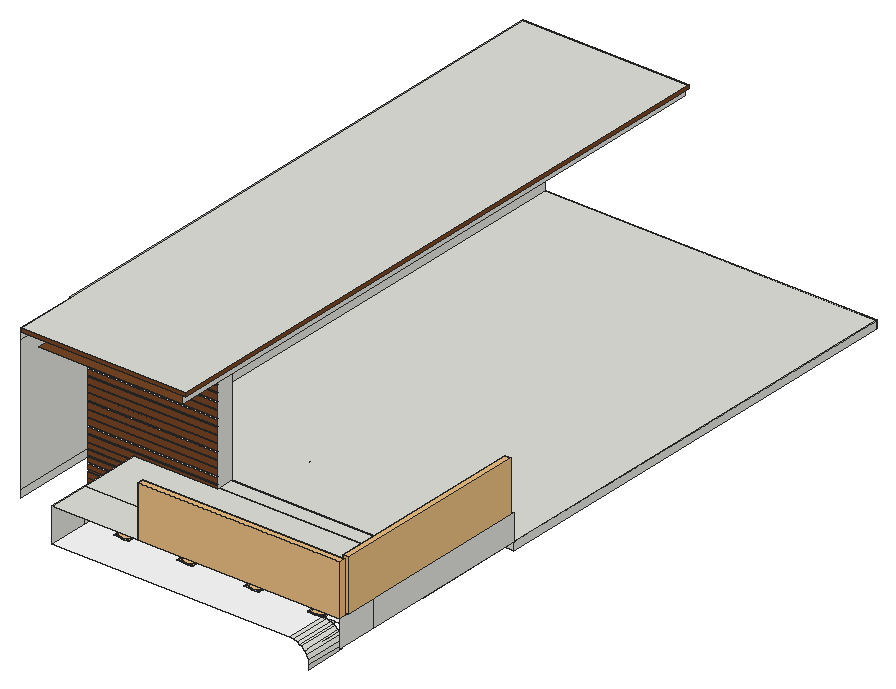
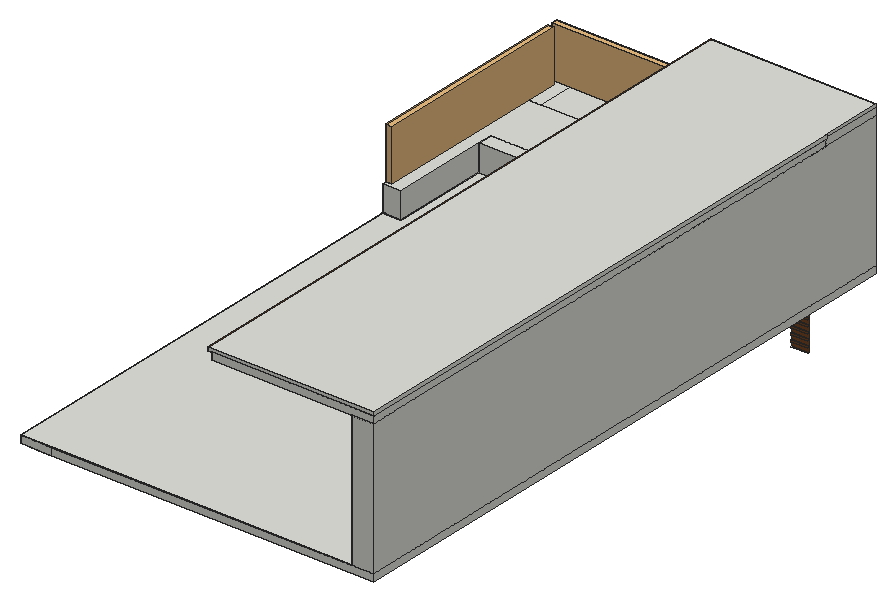
# SketchUp Ruby script. Lengths in inches.
U = 1.inch
M = Sketchup.active_model
def pt(a) = Geom::Point3d.new(a.map { |v| v * U })
def face(e, loops, mat)
  f = e.add_face(loops[0].map { |a| pt(a) })
  loops[1..].each { |l| e.add_face(l.map { |a| pt(a) }).erase! }
  f.material = f.back_material = mat if mat
  f
end
# faces: each face lists its corners as indices into pts; further lists are holes
def faces(e, pts, list, mat = nil) = list.each { |f| face(e, (f[0].is_a?(Array) ? f : [f]).map { |l| l.map { |i| pts[i] } }, mat) }
# xy, xz, yz: faces in a plane at the given z, y or x. An outline is a flat list of corners, or four numbers for a rectangle; further outlines are holes
def ring(l) = l.size == 4 ? [[l[0], l[1]], [l[2], l[1]], [l[2], l[3]], [l[0], l[3]]] : l.each_slice(2).to_a
def flat(e, list, mat, &to3) = list.each { |f| face(e, (f[0].is_a?(Array) ? f : [f]).map { |l| ring(l).map { |u, v| to3.(u, v) } }, mat) }
def xy(e, z, list, mat = nil) = flat(e, list, mat) { |x, y| [x, y, z] }
def xz(e, y, list, mat = nil) = flat(e, list, mat) { |x, z| [x, y, z] }
def yz(e, x, list, mat = nil) = flat(e, list, mat) { |y, z| [x, y, z] }
def lines(e, pts, list) = list.each { |a, b| e.add_line(pt(pts[a]), pt(pts[b])) }
# prism: a flat outline (further loops are holes) pulled along v
def prism(e, loops, v, mat = nil)
  f = face(e, loops, mat); d = Geom::Vector3d.new(v.map { |x| x * U })
  f.pushpull(f.normal.samedirection?(d) ? d.length : -d.length)
end
def box(e, o, s, mat = nil) = prism(e, [[o, [o[0] + s[0], o[1], o[2]], [o[0] + s[0], o[1] + s[1], o[2]], [o[0], o[1] + s[1], o[2]]]], [0, 0, s[2]], mat)
def at(x, y, z, deg = 0) = Geom::Transformation.translation(pt([x, y, z])) * Geom::Transformation.rotation(ORIGIN, Z_AXIS, deg.degrees)
def axes(o, x, y, z) = Geom::Transformation.new([*x, 0, *y, 0, *z, 0, *pt(o).to_a, 1])
def part(name) = M.definitions.add(name)
# library, detail: a bought-in or finely detailed component or shape, given as its bounding box
def library(name, o, s) = part(name).tap { |d| box(d.entities, o, s) }
def detail(e, o, s) = box(e.add_group.entities, o, s)
def put(e, d, t, mat = nil) = e.add_instance(d, t).tap { |i| i.material = mat if mat }
def group(e, t, mat = nil) = e.add_group.tap { |g| g.transformation = t; g.material = mat if mat }.entities
root = M.entities
M.materials.add("[Color M00]").color = [255, 255, 255]
M.materials.add("[Wood Veneer 01]").color = [120, 70, 37]
c1 = library("Group\#12",[-0.5,-0.5,-0.1],[12.57,12.57,0.2])
c2 = library("Group\#13",[-0.5,-0.5,-0.1],[12.57,12.57,0.2])
c3 = library("Group\#14",[-0.5,-0.5,-0.1],[12.57,12.57,0.2])
c4 = library("Group\#15",[-0.5,-0.5,-0.1],[12.57,12.57,0.2])
c5 = library("Glass Railing",[0,0,0],[139.5,4.76,42])
c6 = library("Group\#8",[-0.5,-0.5,-0.1],[8.875,8.875,0.2])
c7 = library("Group\#9",[-0.5,-0.5,-0.1],[8.875,8.875,0.2])
c8 = library("Group\#11",[-0.5,-0.5,-0.1],[8.875,8.875,0.2])
xy(root,277.97,[[404.9375,346.73,445.11,348.1]])
xy(root,278.29,[[338.58,346.73,352.5,348.1]])
xy(root,281.74,[[404.9375,346.73,445.11,348.1]])
xy(root,282.01,[[338.58,346.73,352.5,348.1]])
xy(root,283.15,[[404.9375,346.73,445.11,348.1]])
xy(root,283.42,[[338.58,346.73,352.5,348.1]])
xy(root,286.91,[[404.9375,346.73,445.11,348.1]])
xy(root,287.14,[[338.58,346.73,352.5,348.1]])
xy(root,288.33,[[404.9375,346.73,445.11,348.1]])
xy(root,288.56,[[338.58,346.73,352.5,348.1]])
xy(root,292.09,[[404.9375,346.73,445.11,348.1]])
xy(root,292.28,[[338.58,346.73,352.5,348.1]])
xy(root,293.51,[[404.9375,346.73,445.11,348.1]])
xy(root,293.6875,[[338.58,346.73,352.5,348.1]])
xy(root,296,[[479.29,440.43,567.52,449.58]])
xy(root,297.27,[[404.9375,346.73,445.11,348.1]])
xy(root,297.41,[[338.58,346.73,352.5,348.1]])
xy(root,298.69,[[404.9375,346.73,445.11,348.1]])
xy(root,298.82,[[338.58,346.73,352.5,348.1]])
xy(root,302.45,[[404.9375,346.73,445.11,348.1]])
xy(root,302.54,[[338.58,346.73,352.5,348.1]])
xy(root,303.86,[[404.9375,346.73,445.11,348.1]])
xy(root,303.96,[[338.58,346.73,352.5,348.1]])
xy(root,307.63,[[404.9375,346.73,445.11,348.1]])
xy(root,307.68,[[338.58,346.73,352.5,348.1]])
xy(root,309.04,[[404.9375,346.73,445.11,348.1]])
xy(root,309.09,[[338.58,346.73,352.5,348.1]])
xy(root,312.81,[[338.58,346.73,352.5,348.1],[404.9375,346.73,445.11,348.1],[352.5,348.1,404.9375,354.42]])
xy(root,314.22,[[338.58,346.73,445.11,348.1]])
xy(root,317.66,[[376.54,346.73,445.11,348.1]])
xy(root,319.25,[[588.04,296.73,597.79,348.1],[588.04,348.1,597.79,440.43],[338.58,355.13,338.58,804.07,567.52,804.07,567.52,449.58,432.33,449.58,432.33,355.13],[338.58,355.13,338.58,804.07,567.52,804.07,567.52,449.58,432.33,449.58,432.33,355.13],[586.74,440.43,597.79,811.1],
  [597.79,440.43,612.79,811.1]])
xy(root,319.25,[[[376.54,262.6,376.54,348.1,588.04,348.1,588.04,296.73,571.21,296.73,571.21,262.6],[567.02,295.68,568.5,296.02,569.84,296.73,570.95,297.76,571.76,299.05,572.2,300.5,572.26,302.01,571.92,303.49,571.21,304.83,570.17,305.94,568.89,306.75,567.4375,307.19,565.92,307.25,564.44,306.91,563.1,306.2,561.99,305.16,561.18,303.88,560.74,302.43,560.69,300.91,561.02,299.43,561.74,298.09,562.77,296.98,564.06,296.18,565.51,295.73],[407.66,295.68,409.14,296.02,410.48,296.73,411.59,297.76,412.39,299.05,412.84,300.5,412.89,302.01,412.55,303.49,411.84,304.83,410.81,305.94,409.52,306.75,408.07,307.19,406.56,307.25,405.08,306.91,403.74,306.2,402.625,305.16,401.82,303.88,401.375,302.43,401.32,300.91,401.66,299.43,402.37,298.09,403.41,296.98,404.69,296.18,406.14,295.73],[459.85,295.68,461.32,296.02,462.66,296.73,463.78,297.76,464.58,299.05,465.03,300.5,465.08,302.01,464.74,303.49,464.03,304.83,463,305.94,461.71,306.75,460.26,307.19,458.74,307.25,457.26,306.91,455.92,306.2,454.8125,305.16,454.01,303.88,453.5625,302.43,453.51,300.91,453.85,299.43,454.56,298.09,455.59,296.98,456.88,296.18,458.33,295.73],[514.22,295.68,515.7,296.02,517.04,296.73,518.15,297.76,518.96,299.05,519.4,300.5,519.46,302.01,519.12,303.49,518.4,304.83,517.37,305.94,516.08,306.75,514.63,307.19,513.12,307.25,511.64,306.91,510.3,306.2,509.1875,305.16,508.38,303.88,507.9375,302.43,507.88,300.91,508.22,299.43,508.93,298.09,509.97,296.98,511.25,296.18,512.7,295.73]],[445.11,348.1,588.04,440.43]],"[Color M00]")
xy(root,321.49,[[338.58,346.73,376.54,348.1]])
xy(root,324.09,[[338.58,346.73,376.54,348.1]])
xy(root,325.25,[[445.11,348.1,597.79,440.43],[597.79,348.1,612.79,440.43]])
xy(root,325.375,[[341.61,360.71,597.79,360.71,597.79,440.43,612.79,440.43,612.79,811.1,341.61,811.1]])
xy(root,327.93,[[338.58,346.73,376.54,348.1]])
xy(root,329.07,[[338.58,346.73,376.54,348.1]])
xy(root,332.9,[[338.58,346.73,376.54,348.1]])
xy(root,334.04,[[338.58,346.73,376.54,348.1]])
xy(root,337.875,[[338.58,346.73,376.54,348.1]])
xy(root,339.02,[[338.58,346.73,376.54,348.1]])
xy(root,342.85,[[338.58,346.73,376.54,348.1]])
xy(root,343.99,[[338.58,346.73,376.54,348.1]])
xy(root,346.9375,[[376.54,262.6,597.79,296.73],[597.79,262.6,612.67,296.73],[376.54,296.73,612.79,296.73,612.79,440.43,597.79,440.43,597.79,348.1,445.11,348.1,445.11,346.73,376.54,346.73],[376.54,346.73,445.11,348.1],[445.11,348.1,597.79,360.71]])
xy(root,349.02,[[338.58,346.73,376.54,348.1],[376.54,346.73,445.11,348.1]])
xy(root,350.07,[[338.58,346.73,445.11,348.1]])
xy(root,355.09,[[338.58,346.73,376.54,348.1],[376.54,346.73,445.11,348.1]])
xy(root,356.14,[[338.58,346.73,445.11,348.1]])
xy(root,361.17,[[338.58,346.73,376.54,348.1],[376.54,346.73,445.11,348.1]])
xy(root,362.21,[[338.58,346.73,445.11,348.1]])
xy(root,367.24,[[338.58,346.73,376.54,348.1],[376.54,346.73,445.11,348.1]])
xy(root,368.29,[[338.58,346.73,445.11,348.1]])
xy(root,373.32,[[338.58,346.73,376.54,348.1],[376.54,346.73,445.11,348.1]])
xy(root,374.36,[[338.58,346.73,445.11,348.1]])
xy(root,379.39,[[338.58,346.73,376.54,348.1],[376.54,346.73,445.11,348.1]])
xy(root,380.4375,[[338.58,346.73,445.11,348.1]])
xy(root,385.46,[[338.58,346.73,376.54,348.1],[376.54,346.73,445.11,348.1]])
xy(root,386.51,[[338.58,346.73,445.11,348.1]])
xy(root,391.54,[[338.58,346.73,376.54,348.1],[376.54,346.73,445.11,348.1]])
xy(root,392.59,[[338.58,346.73,445.11,348.1]])
xy(root,397.61,[[338.58,346.73,376.54,348.1],[376.54,346.73,445.11,348.1]])
xy(root,398.66,[[338.58,346.73,445.11,348.1]])
xy(root,403.6875,[[338.58,346.73,376.54,348.1],[376.54,346.73,445.11,348.1]])
xy(root,404.97,[[338.58,346.73,445.11,348.1]])
xy(root,410,[[338.58,346.73,376.54,348.1],[376.54,346.73,445.11,348.1]])
xy(root,411.28,[[338.58,346.73,445.11,348.1]])
xy(root,416.3125,[[338.58,346.73,376.54,348.1],[376.54,346.73,445.11,348.1]])
xy(root,417.6,[[338.58,346.73,445.11,348.1]])
xy(root,422.625,[[338.58,346.73,376.54,348.1],[376.54,346.73,445.11,348.1]])
xy(root,423.91,[[338.58,346.73,445.11,348.1]])
xy(root,428.9375,[[338.58,346.73,376.54,348.1],[376.54,346.73,445.11,348.1]])
xy(root,430.22,[[338.58,346.73,445.11,348.1]])
xy(root,435.25,[[338.58,346.73,376.54,346.73,376.54,360.71,341.61,360.71,341.61,811.1,338.58,811.1],[376.54,346.73,445.11,360.71],[323.43,348.1,338.58,811.1],[341.61,360.71,376.54,811.1]])
xy(root,435.25,[[[338.58,296.73,338.58,346.73,445.11,346.73,445.11,360.71,376.54,360.71,376.54,811.1,456.36,811.1,456.36,296.73],[397,314.77,398.02,314.91,398.97,315.3,399.79,315.93,400.41,316.74,400.81,317.69,400.94,318.71,400.81,319.73,400.41,320.68,399.79,321.49,398.97,322.12,398.02,322.51,397,322.65,395.99,322.51,395.04,322.12,394.22,321.49,393.59,320.68,393.2,319.73,393.07,318.71,393.2,317.69,393.59,316.74,394.22,315.93,395.04,315.3,395.99,314.91],[443,314.77,444.02,314.91,444.97,315.3,445.79,315.93,446.41,316.74,446.81,317.69,446.94,318.71,446.81,319.73,446.41,320.68,445.79,321.49,444.97,322.12,444.02,322.51,443,322.65,441.99,322.51,441.04,322.12,440.22,321.49,439.59,320.68,439.2,319.73,439.07,318.71,439.2,317.69,439.59,316.74,440.22,315.93,441.04,315.3,441.99,314.91],[355.25,314.77,356.27,314.91,357.22,315.3,358.04,315.93,358.66,316.74,359.06,317.69,359.19,318.71,359.06,319.73,358.66,320.68,358.04,321.49,357.22,322.12,356.27,322.51,355.25,322.65,354.24,322.51,353.29,322.12,352.47,321.49,351.84,320.68,351.45,319.73,351.32,318.71,351.45,317.69,351.84,316.74,352.47,315.93,353.29,315.3,354.24,314.91]]],"[Wood Veneer 01]")
xy(root,441.25,[[323.43,296.73,456.36,811.1],[323.18,348.1,323.43,811.1]])
xy(root,441.25,[[456.36,296.73,458.99,811.1]],"[Wood Veneer 01]")
xy(root,443.8125,[[323.43,296.73,458.99,296.73,458.99,811.1,323.18,811.1,323.18,348.1,323.43,348.1]])
xz(root,296.73,[[579.8,316.65,577.86,317.8,574.62,318.88,571.21,319.25,579.8,319.25],[597.79,325.25,612.67,346.9375]])
xz(root,296.73,[[323.43,441.25,458.99,443.8125]],"[Wood Veneer 01]")
xz(root,346.73,[[404.9375,277.97,445.11,281.74],[338.58,278.29,352.5,282.01],[404.9375,283.15,445.11,286.91],[338.58,283.42,352.5,287.14],[404.9375,288.33,445.11,292.09],
  [338.58,288.56,352.5,292.28],[404.9375,293.51,445.11,297.27],[338.58,293.6875,352.5,297.41],[404.9375,298.69,445.11,302.45],[338.58,298.82,352.5,302.54],
  [404.9375,303.86,445.11,307.63],[338.58,303.96,352.5,307.68],[404.9375,309.04,445.11,312.81],[338.58,309.09,352.5,312.81],[338.58,314.22,445.11,317.66],
  [338.58,317.66,376.54,321.49],[338.58,324.09,376.54,327.93],[338.58,329.07,376.54,332.9],[338.58,334.04,376.54,337.875],[338.58,339.02,376.54,342.85],
  [338.58,343.99,376.54,343.99,376.54,346.9375,445.11,346.9375,445.11,349.02,338.58,349.02],[338.58,350.07,445.11,355.09],[338.58,356.14,445.11,361.17],[338.58,362.21,445.11,367.24],[338.58,368.29,445.11,373.32],
  [338.58,374.36,445.11,379.39],[338.58,380.4375,445.11,385.46],[338.58,386.51,445.11,391.54],[338.58,392.59,445.11,397.61],[338.58,398.66,445.11,403.6875],
  [338.58,404.97,445.11,410],[338.58,411.28,445.11,416.3125],[338.58,417.6,445.11,422.625],[338.58,423.91,445.11,428.9375],[338.58,430.22,445.11,435.25]],"[Wood Veneer 01]")
xz(root,348.1,[[404.9375,277.97,445.11,281.74],[404.9375,283.15,445.11,286.91],[404.9375,288.33,445.11,292.09],[404.9375,293.51,445.11,297.27],[376.54,319.25,445.11,343.99],
  [445.11,325.25,597.79,346.9375],[376.54,343.99,445.11,346.9375],[323.18,441.25,323.43,443.8125]])
xz(root,348.1,[[404.9375,281.74,445.11,283.15],[338.58,282.01,352.5,283.42],[404.9375,286.91,445.11,288.33],[338.58,287.14,352.5,288.56],[404.9375,292.09,445.11,293.51],
  [338.58,292.28,352.5,293.6875],[404.9375,297.27,445.11,298.69],[338.58,297.41,352.5,298.82],[404.9375,302.45,445.11,303.86],[338.58,302.54,352.5,303.96],
  [404.9375,307.63,445.11,309.04],[338.58,307.68,352.5,309.09],[338.58,312.81,445.11,314.22],[376.54,317.66,445.11,317.66,445.11,319.25,597.79,319.25,597.79,325.25,445.11,325.25,445.11,319.25,376.54,319.25],[338.58,321.49,376.54,324.09],
  [338.58,327.93,376.54,329.07],[338.58,332.9,376.54,334.04],[338.58,337.875,376.54,339.02],[338.58,342.85,376.54,343.99],[338.58,349.02,445.11,350.07],
  [338.58,355.09,445.11,356.14],[338.58,361.17,445.11,362.21],[338.58,367.24,445.11,368.29],[338.58,373.32,445.11,374.36],[338.58,379.39,445.11,380.4375],
  [338.58,385.46,445.11,386.51],[338.58,391.54,445.11,392.59],[338.58,397.61,445.11,398.66],[338.58,403.6875,445.11,404.97],[338.58,410,445.11,411.28],
  [338.58,416.3125,445.11,417.6],[338.58,422.625,445.11,423.91],[338.58,428.9375,445.11,430.22]],"[Wood Veneer 01]")
xz(root,360.71,[[341.61,325.375,341.61,435.25,445.11,435.25,445.11,346.9375,597.79,346.9375,597.79,325.375]])
xz(root,440.43,[[597.79,319.25,612.79,325.25],[597.79,325.25,612.79,325.375],[597.79,325.375,612.79,346.9375]])
xz(root,811.1,[[323.43,319.25,586.74,325.25],[586.74,319.25,612.79,325.25],[323.43,325.25,323.43,435.25,341.61,435.25,341.61,325.375,586.74,325.375,586.74,325.25],[586.74,325.25,612.79,325.375],[323.43,435.25,456.36,441.25],
  [323.18,441.25,458.99,443.8125]])
yz(root,323.18,[[348.1,441.25,811.1,443.8125]])
yz(root,323.43,[[296.73,319.25,811.1,325.25],[296.73,325.25,811.1,435.25],[296.73,435.25,348.1,441.25],[348.1,435.25,811.1,441.25],[296.73,441.25,348.1,443.8125]])
yz(root,341.61,[[360.71,325.375,811.1,435.25]])
yz(root,376.54,[[346.73,317.66,348.1,319.25],[262.6,319.25,296.73,346.9375],[296.73,319.25,296.73,346.9375,346.73,346.9375,346.73,343.99,348.1,343.99,348.1,342.85,346.73,342.85,346.73,339.02,348.1,339.02,348.1,337.875,346.73,337.875,346.73,334.04,348.1,334.04,348.1,332.9,346.73,332.9,346.73,329.07,348.1,329.07,348.1,327.93,346.73,327.93,346.73,324.09,348.1,324.09,348.1,321.49,346.73,321.49,346.73,319.25],[346.73,319.25,348.1,321.49],[346.73,324.09,348.1,327.93],
  [346.73,329.07,348.1,332.9],[346.73,334.04,348.1,337.875],[346.73,339.02,348.1,342.85],[346.73,343.99,348.1,346.9375]])
yz(root,404.9375,[[346.73,277.97,348.1,281.74],[346.73,283.15,348.1,286.91],[346.73,288.33,348.1,292.09],[346.73,293.51,348.1,297.27]])
yz(root,445.11,[[346.73,277.97,348.1,281.74],[346.73,283.15,348.1,286.91],[346.73,288.33,348.1,292.09],[346.73,293.51,348.1,297.27],[346.73,346.9375,360.71,346.9375,360.71,435.25,346.73,435.25,346.73,430.22,348.1,430.22,348.1,428.9375,346.73,428.9375,346.73,423.91,348.1,423.91,348.1,422.625,346.73,422.625,346.73,417.6,348.1,417.6,348.1,416.3125,346.73,416.3125,346.73,411.28,348.1,411.28,348.1,410,346.73,410,346.73,404.97,348.1,404.97,348.1,403.6875,346.73,403.6875,346.73,398.66,348.1,398.66,348.1,397.61,346.73,397.61,346.73,392.59,348.1,392.59,348.1,391.54,346.73,391.54,346.73,386.51,348.1,386.51,348.1,385.46,346.73,385.46,346.73,380.4375,348.1,380.4375,348.1,379.39,346.73,379.39,346.73,374.36,348.1,374.36,348.1,373.32,346.73,373.32,346.73,368.29,348.1,368.29,348.1,367.24,346.73,367.24,346.73,362.21,348.1,362.21,348.1,361.17,346.73,361.17,346.73,356.14,348.1,356.14,348.1,355.09,346.73,355.09,346.73,350.07,348.1,350.07,348.1,349.02,346.73,349.02]])
yz(root,456.36,[[296.73,435.25,811.1,441.25]])
yz(root,458.99,[[296.73,441.25,811.1,443.8125]],"[Wood Veneer 01]")
yz(root,597.79,[[348.1,319.25,440.43,325.25],[348.1,325.25,348.1,346.9375,360.71,346.9375,360.71,325.375,440.43,325.375,440.43,325.25],[360.71,325.375,440.43,346.9375]])
yz(root,612.67,[[262.6,325.25,296.73,346.9375]])
yz(root,612.79,[[440.43,319.25,811.1,325.25],[296.73,325.25,440.43,346.9375],[440.43,325.25,811.1,325.375]])
p = [[587.03,262.6,300.95],[587.16,262.6,304.37],[587.16,296.73,304.37],[587.03,296.73,300.95],[586.56,262.6,307.74],[586.56,296.73,307.74],
  [585.26,262.6,310.9],[585.26,296.73,310.9],[583.31,262.6,313.72],[583.31,296.73,313.72],[580.81,262.6,316.05],[580.81,296.73,316.05],
  [579.8,262.6,316.65],[579.8,296.73,316.65],[577.86,262.6,317.8],[577.86,296.73,317.8],[574.62,262.6,318.88],[574.62,296.73,318.88],
  [571.21,262.6,319.25],[571.21,296.73,319.25],[406.14,295.73,319.25],[404.69,296.18,319.25],[404.69,296.18,320],[406.14,295.73,320],
  [407.66,295.68,319.25],[407.66,295.68,320],[409.14,296.02,319.25],[409.14,296.02,320],[458.33,295.73,319.25],[456.88,296.18,319.25],
  [456.88,296.18,320],[458.33,295.73,320],[459.85,295.68,319.25],[459.85,295.68,320],[461.32,296.02,319.25],[461.32,296.02,320],
  [512.7,295.73,319.25],[511.25,296.18,319.25],[511.25,296.18,320],[512.7,295.73,320],[514.22,295.68,319.25],[514.22,295.68,320],
  [515.7,296.02,319.25],[515.7,296.02,320],[565.51,295.73,319.25],[564.06,296.18,319.25],[564.06,296.18,320],[565.51,295.73,320],
  [567.02,295.68,319.25],[567.02,295.68,320],[568.5,296.02,319.25],[568.5,296.02,320],[410.48,296.73,319.25],[410.48,296.73,320],
  [462.66,296.73,319.25],[462.66,296.73,320],[517.04,296.73,319.25],[517.04,296.73,320],[569.84,296.73,319.25],[569.84,296.73,320],
  [403.41,296.98,319.25],[403.41,296.98,320],[455.59,296.98,319.25],[455.59,296.98,320],[509.97,296.98,319.25],[509.97,296.98,320],
  [562.77,296.98,319.25],[562.77,296.98,320],[411.59,297.76,319.25],[411.59,297.76,320],[463.78,297.76,319.25],[463.78,297.76,320],
  [518.15,297.76,319.25],[518.15,297.76,320],[570.95,297.76,319.25],[570.95,297.76,320],[402.37,298.09,319.25],[402.37,298.09,320],
  [454.56,298.09,319.25],[454.56,298.09,320],[508.93,298.09,319.25],[508.93,298.09,320],[561.74,298.09,319.25],[561.74,298.09,320],
  [412.39,299.05,319.25],[412.39,299.05,320],[464.58,299.05,319.25],[464.58,299.05,320],[518.96,299.05,319.25],[518.96,299.05,320],
  [571.76,299.05,319.25],[571.76,299.05,320],[401.66,299.43,319.25],[401.66,299.43,320],[453.85,299.43,319.25],[453.85,299.43,320],
  [508.22,299.43,319.25],[508.22,299.43,320],[561.02,299.43,319.25],[561.02,299.43,320],[412.84,300.5,319.25],[412.84,300.5,320],
  [465.03,300.5,319.25],[465.03,300.5,320],[519.4,300.5,319.25],[519.4,300.5,320],[572.2,300.5,319.25],[572.2,300.5,320],
  [401.32,300.91,319.25],[401.32,300.91,320],[453.51,300.91,319.25],[453.51,300.91,320],[507.88,300.91,319.25],[507.88,300.91,320],
  [560.69,300.91,319.25],[560.69,300.91,320],[412.89,302.01,319.25],[412.89,302.01,320],[465.08,302.01,319.25],[465.08,302.01,320],
  [519.46,302.01,319.25],[519.46,302.01,320],[572.26,302.01,319.25],[572.26,302.01,320],[401.375,302.43,319.25],[401.375,302.43,320],
  [453.5625,302.43,319.25],[453.5625,302.43,320],[507.9375,302.43,319.25],[507.9375,302.43,320],[560.74,302.43,319.25],[560.74,302.43,320],
  [412.55,303.49,319.25],[412.55,303.49,320],[464.74,303.49,319.25],[464.74,303.49,320],[519.12,303.49,319.25],[519.12,303.49,320],
  [571.92,303.49,319.25],[571.92,303.49,320],[401.82,303.88,319.25],[401.82,303.88,320],[454.01,303.88,319.25],[454.01,303.88,320],
  [508.38,303.88,319.25],[508.38,303.88,320],[561.18,303.88,319.25],[561.18,303.88,320],[411.84,304.83,319.25],[411.84,304.83,320],
  [464.03,304.83,319.25],[464.03,304.83,320],[518.4,304.83,319.25],[518.4,304.83,320],[571.21,304.83,319.25],[571.21,304.83,320],
  [402.625,305.16,319.25],[402.625,305.16,320],[454.8125,305.16,319.25],[454.8125,305.16,320],[509.1875,305.16,319.25],[509.1875,305.16,320],
  [561.99,305.16,319.25],[561.99,305.16,320],[410.81,305.94,319.25],[410.81,305.94,320],[463,305.94,319.25],[463,305.94,320],
  [517.37,305.94,319.25],[517.37,305.94,320],[570.17,305.94,319.25],[570.17,305.94,320],[403.74,306.2,319.25],[403.74,306.2,320],
  [455.92,306.2,319.25],[455.92,306.2,320],[510.3,306.2,319.25],[510.3,306.2,320],[563.1,306.2,319.25],[563.1,306.2,320],
  [409.52,306.75,319.25],[409.52,306.75,320],[461.71,306.75,319.25],[461.71,306.75,320],[516.08,306.75,319.25],[516.08,306.75,320],
  [568.89,306.75,319.25],[568.89,306.75,320],[405.08,306.91,319.25],[405.08,306.91,320],[457.26,306.91,319.25],[457.26,306.91,320],
  [511.64,306.91,319.25],[511.64,306.91,320],[564.44,306.91,319.25],[564.44,306.91,320],[408.07,307.19,319.25],[408.07,307.19,320],
  [460.26,307.19,319.25],[460.26,307.19,320],[514.63,307.19,319.25],[514.63,307.19,320],[567.4375,307.19,319.25],[567.4375,307.19,320],
  [406.56,307.25,319.25],[406.56,307.25,320],[458.74,307.25,319.25],[458.74,307.25,320],[513.12,307.25,319.25],[513.12,307.25,320],
  [565.92,307.25,319.25],[565.92,307.25,320],[355.25,314.77,435.25],[354.24,314.91,435.25],[354.24,314.91,435.875],[355.25,314.77,435.875],
  [356.27,314.91,435.25],[356.27,314.91,435.875],[397,314.77,435.25],[395.99,314.91,435.25],[395.99,314.91,435.875],[397,314.77,435.875],
  [398.02,314.91,435.25],[398.02,314.91,435.875],[443,314.77,435.25],[441.99,314.91,435.25],[441.99,314.91,435.875],[443,314.77,435.875],
  [444.02,314.91,435.25],[444.02,314.91,435.875],[353.29,315.3,435.25],[353.29,315.3,435.875],[357.22,315.3,435.25],[357.22,315.3,435.875],
  [395.04,315.3,435.25],[395.04,315.3,435.875],[398.97,315.3,435.25],[398.97,315.3,435.875],[441.04,315.3,435.25],[441.04,315.3,435.875],
  [444.97,315.3,435.25],[444.97,315.3,435.875],[352.47,315.93,435.25],[352.47,315.93,435.875],[358.04,315.93,435.25],[358.04,315.93,435.875],
  [394.22,315.93,435.25],[394.22,315.93,435.875],[399.79,315.93,435.25],[399.79,315.93,435.875],[440.22,315.93,435.25],[440.22,315.93,435.875],
  [445.79,315.93,435.25],[445.79,315.93,435.875],[351.84,316.74,435.25],[351.84,316.74,435.875],[358.66,316.74,435.25],[358.66,316.74,435.875],
  [393.59,316.74,435.25],[393.59,316.74,435.875],[400.41,316.74,435.25],[400.41,316.74,435.875],[439.59,316.74,435.25],[439.59,316.74,435.875],
  [446.41,316.74,435.25],[446.41,316.74,435.875],[351.45,317.69,435.25],[351.45,317.69,435.875],[359.06,317.69,435.25],[359.06,317.69,435.875],
  [393.2,317.69,435.25],[393.2,317.69,435.875],[400.81,317.69,435.25],[400.81,317.69,435.875],[439.2,317.69,435.25],[439.2,317.69,435.875],
  [446.81,317.69,435.25],[446.81,317.69,435.875],[351.32,318.71,435.25],[351.32,318.71,435.875],[359.19,318.71,435.25],[359.19,318.71,435.875],
  [393.07,318.71,435.25],[393.07,318.71,435.875],[400.94,318.71,435.25],[400.94,318.71,435.875],[439.07,318.71,435.25],[439.07,318.71,435.875],
  [446.94,318.71,435.25],[446.94,318.71,435.875],[351.45,319.73,435.25],[351.45,319.73,435.875],[359.06,319.73,435.25],[359.06,319.73,435.875],
  [393.2,319.73,435.25],[393.2,319.73,435.875],[400.81,319.73,435.25],[400.81,319.73,435.875],[439.2,319.73,435.25],[439.2,319.73,435.875],
  [446.81,319.73,435.25],[446.81,319.73,435.875],[351.84,320.68,435.25],[351.84,320.68,435.875],[358.66,320.68,435.25],[358.66,320.68,435.875],
  [393.59,320.68,435.25],[393.59,320.68,435.875],[400.41,320.68,435.25],[400.41,320.68,435.875],[439.59,320.68,435.25],[439.59,320.68,435.875],
  [446.41,320.68,435.25],[446.41,320.68,435.875],[352.47,321.49,435.25],[352.47,321.49,435.875],[358.04,321.49,435.25],[358.04,321.49,435.875],
  [394.22,321.49,435.25],[394.22,321.49,435.875],[399.79,321.49,435.25],[399.79,321.49,435.875],[440.22,321.49,435.25],[440.22,321.49,435.875],
  [445.79,321.49,435.25],[445.79,321.49,435.875],[353.29,322.12,435.25],[353.29,322.12,435.875],[357.22,322.12,435.25],[357.22,322.12,435.875],
  [395.04,322.12,435.25],[395.04,322.12,435.875],[398.97,322.12,435.25],[398.97,322.12,435.875],[441.04,322.12,435.25],[441.04,322.12,435.875],
  [444.97,322.12,435.25],[444.97,322.12,435.875],[354.24,322.51,435.25],[354.24,322.51,435.875],[356.27,322.51,435.25],[356.27,322.51,435.875],
  [395.99,322.51,435.25],[395.99,322.51,435.875],[398.02,322.51,435.25],[398.02,322.51,435.875],[441.99,322.51,435.25],[441.99,322.51,435.875],
  [444.02,322.51,435.25],[444.02,322.51,435.875],[355.25,322.65,435.25],[355.25,322.65,435.875],[397,322.65,435.25],[397,322.65,435.875],
  [443,322.65,435.25],[443,322.65,435.875],[432.33,355.13,319.25],[432.33,348.1,319.25],[338.58,355.13,319.25],[338.58,348.1,319.25],
  [597.79,296.73,325.25],[597.79,262.6,325.25]]
faces(root,p,[[0,1,2,3],[1,4,5,2],[4,6,7,5],[6,8,9,7],[8,10,11,9],[10,12,13,11],[12,14,15,13],[14,16,17,15],
  [16,18,19,17],[20,21,22,23],[24,20,23,25],[26,24,25,27],[28,29,30,31],[32,28,31,33],[34,32,33,35],[36,37,38,39],
  [40,36,39,41],[42,40,41,43],[44,45,46,47],[48,44,47,49],[50,48,49,51],[52,26,27,53],[54,34,35,55],[56,42,43,57],
  [58,50,51,59],[21,60,61,22],[29,62,63,30],[37,64,65,38],[45,66,67,46],[68,52,53,69],[70,54,55,71],[72,56,57,73],
  [74,58,59,75],[60,76,77,61],[62,78,79,63],[64,80,81,65],[66,82,83,67],[84,68,69,85],[86,70,71,87],[88,72,73,89],
  [90,74,75,91],[76,92,93,77],[78,94,95,79],[80,96,97,81],[82,98,99,83],[100,84,85,101],[102,86,87,103],[104,88,89,105],
  [106,90,91,107],[92,108,109,93],[94,110,111,95],[96,112,113,97],[98,114,115,99],[116,100,101,117],[118,102,103,119],[120,104,105,121],
  [122,106,107,123],[108,124,125,109],[110,126,127,111],[112,128,129,113],[114,130,131,115],[132,116,117,133],[134,118,119,135],[136,120,121,137],
  [138,122,123,139],[124,140,141,125],[126,142,143,127],[128,144,145,129],[130,146,147,131],[148,132,133,149],[150,134,135,151],[152,136,137,153],
  [154,138,139,155],[140,156,157,141],[142,158,159,143],[144,160,161,145],[146,162,163,147],[164,148,149,165],[166,150,151,167],[168,152,153,169],
  [170,154,155,171],[156,172,173,157],[158,174,175,159],[160,176,177,161],[162,178,179,163],[180,164,165,181],[182,166,167,183],[184,168,169,185],
  [186,170,171,187],[172,188,189,173],[174,190,191,175],[176,192,193,177],[178,194,195,179],[196,180,181,197],[198,182,183,199],[200,184,185,201],
  [202,186,187,203],[188,204,205,189],[190,206,207,191],[192,208,209,193],[194,210,211,195],[204,196,197,205],[206,198,199,207],[208,200,201,209],
  [210,202,203,211]])
faces(root,p,[[212,213,214,215],[216,212,215,217],[218,219,220,221],[222,218,221,223],[224,225,226,227],[228,224,227,229],[213,230,231,214],[232,216,217,233],
  [219,234,235,220],[236,222,223,237],[225,238,239,226],[240,228,229,241],[230,242,243,231],[244,232,233,245],[234,246,247,235],[248,236,237,249],
  [238,250,251,239],[252,240,241,253],[242,254,255,243],[256,244,245,257],[246,258,259,247],[260,248,249,261],[250,262,263,251],[264,252,253,265],
  [254,266,267,255],[268,256,257,269],[258,270,271,259],[272,260,261,273],[262,274,275,263],[276,264,265,277],[266,278,279,267],[280,268,269,281],
  [270,282,283,271],[284,272,273,285],[274,286,287,275],[288,276,277,289],[278,290,291,279],[292,280,281,293],[282,294,295,283],[296,284,285,297],
  [286,298,299,287],[300,288,289,301],[290,302,303,291],[304,292,293,305],[294,306,307,295],[308,296,297,309],[298,310,311,299],[312,300,301,313],
  [302,314,315,303],[316,304,305,317],[306,318,319,307],[320,308,309,321],[310,322,323,311],[324,312,313,325],[314,326,327,315],[328,316,317,329],
  [318,330,331,319],[332,320,321,333],[322,334,335,323],[336,324,325,337],[326,338,339,327],[340,328,329,341],[330,342,343,331],[344,332,333,345],
  [334,346,347,335],[348,336,337,349],[338,350,351,339],[350,340,341,351],[342,352,353,343],[352,344,345,353],[346,354,355,347],[354,348,349,355]],"[Wood Veneer 01]")
lines(root,p,[[356,357],[358,359],[360,361]])
put(root,c1,at(401.32,295.68,320))
put(root,c2,at(453.51,295.68,320))
put(root,c3,at(507.88,295.68,320))
put(root,c4,at(560.69,295.68,320))
put(root,c5,axes([447.02,262.6,346.9375],[1.18744,0,0],[0,1,0],[0,0,1]))
put(root,c5,axes([612.67,271.06,346.9375],[0,1.18744,0],[-1,0,0],[0,0,1]))
put(root,c6,at(351.32,314.77,435.875))
put(root,c7,at(393.07,314.77,435.875))
put(root,c8,at(439.07,314.77,435.875))
